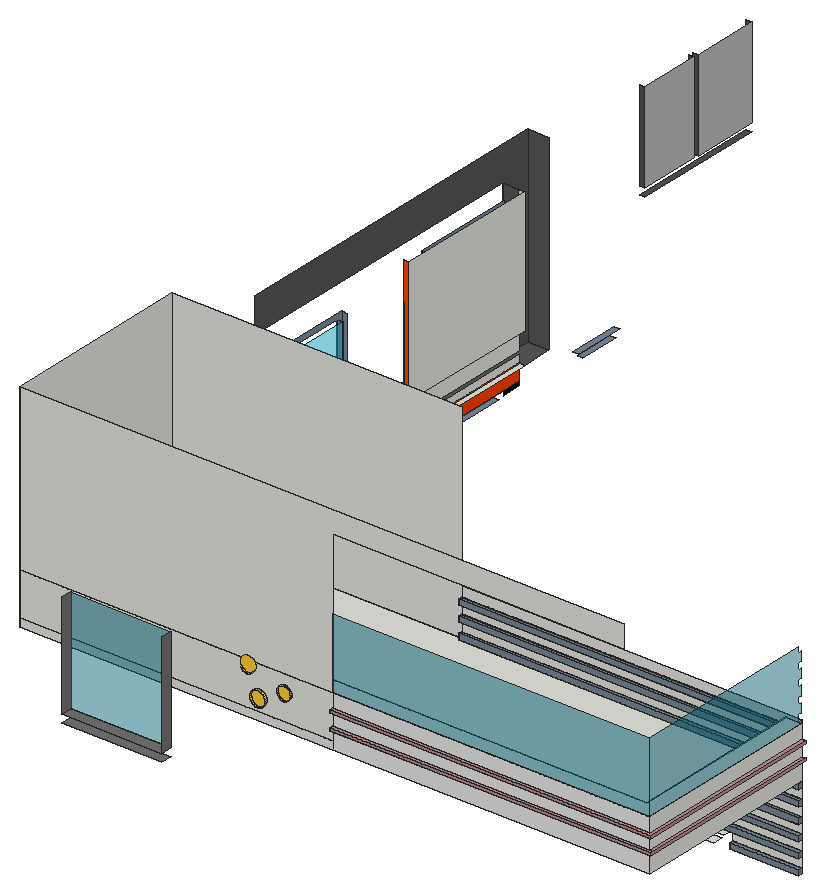
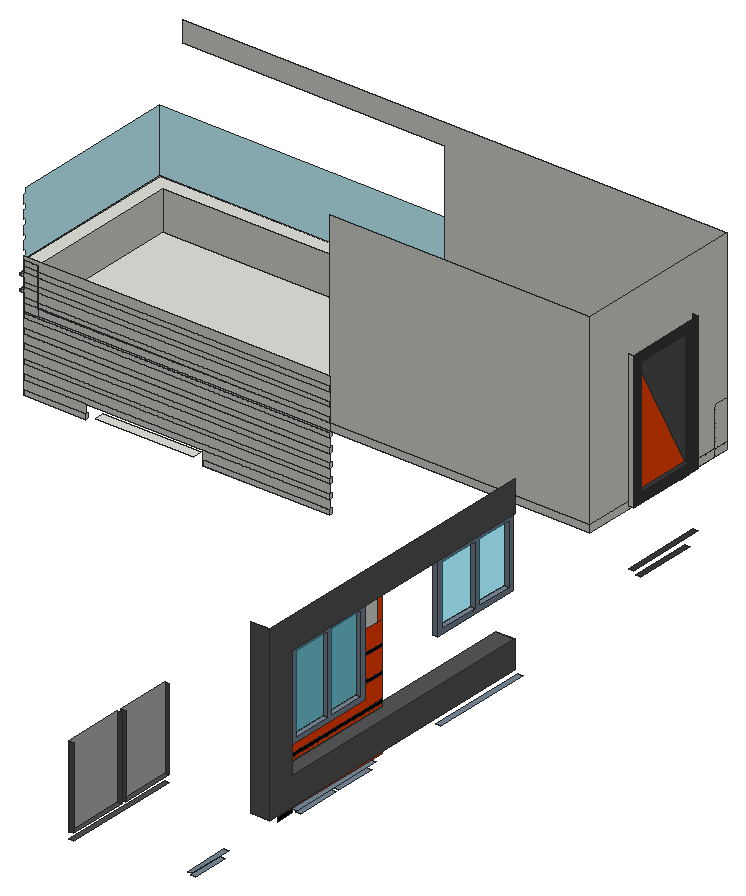
# SketchUp Ruby script. Lengths in inches.
U = 1.inch
M = Sketchup.active_model
def pt(a) = Geom::Point3d.new(a.map { |v| v * U })
def face(e, loops, mat)
  f = e.add_face(loops[0].map { |a| pt(a) })
  loops[1..].each { |l| e.add_face(l.map { |a| pt(a) }).erase! }
  f.material = f.back_material = mat if mat
  f
end
# faces: each face lists its corners as indices into pts; further lists are holes
def faces(e, pts, list, mat = nil) = list.each { |f| face(e, (f[0].is_a?(Array) ? f : [f]).map { |l| l.map { |i| pts[i] } }, mat) }
# xy, xz, yz: faces in a plane at the given z, y or x. An outline is a flat list of corners, or four numbers for a rectangle; further outlines are holes
def ring(l) = l.size == 4 ? [[l[0], l[1]], [l[2], l[1]], [l[2], l[3]], [l[0], l[3]]] : l.each_slice(2).to_a
def flat(e, list, mat, &to3) = list.each { |f| face(e, (f[0].is_a?(Array) ? f : [f]).map { |l| ring(l).map { |u, v| to3.(u, v) } }, mat) }
def xy(e, z, list, mat = nil) = flat(e, list, mat) { |x, y| [x, y, z] }
def xz(e, y, list, mat = nil) = flat(e, list, mat) { |x, z| [x, y, z] }
def yz(e, x, list, mat = nil) = flat(e, list, mat) { |y, z| [x, y, z] }
def lines(e, pts, list) = list.each { |a, b| e.add_line(pt(pts[a]), pt(pts[b])) }
# prism: a flat outline (further loops are holes) pulled along v
def prism(e, loops, v, mat = nil)
  f = face(e, loops, mat); d = Geom::Vector3d.new(v.map { |x| x * U })
  f.pushpull(f.normal.samedirection?(d) ? d.length : -d.length)
end
def box(e, o, s, mat = nil) = prism(e, [[o, [o[0] + s[0], o[1], o[2]], [o[0] + s[0], o[1] + s[1], o[2]], [o[0], o[1] + s[1], o[2]]]], [0, 0, s[2]], mat)
def at(x, y, z, deg = 0) = Geom::Transformation.translation(pt([x, y, z])) * Geom::Transformation.rotation(ORIGIN, Z_AXIS, deg.degrees)
def axes(o, x, y, z) = Geom::Transformation.new([*x, 0, *y, 0, *z, 0, *pt(o).to_a, 1])
def part(name) = M.definitions.add(name)
# library, detail: a bought-in or finely detailed component or shape, given as its bounding box
def library(name, o, s) = part(name).tap { |d| box(d.entities, o, s) }
def detail(e, o, s) = box(e.add_group.entities, o, s)
def put(e, d, t, mat = nil) = e.add_instance(d, t).tap { |i| i.material = mat if mat }
def group(e, t, mat = nil) = e.add_group.tap { |g| g.transformation = t; g.material = mat if mat }.entities
root = M.entities
M.materials.add("[0024_OrangeRed]").color = [255, 69, 0]
M.materials.add("[0110_LightSlateGray]").color = [119, 136, 153]
M.materials.add("[0119_RosyBrown]").color = [188, 143, 143]
M.materials.add("[0135_DarkGray]").color = [81, 81, 81]
M.materials.add("[Color B05]").color = [255, 63, 0]
M.materials.add("[Color D04]").color = [255, 204, 50]
M.materials.add("[Color M05]").color = [114, 114, 114]
M.materials.add("[Color M06]").color = [86, 86, 86]
M.materials.add("[Color M07]").color = [58, 58, 58]
M.materials.add("[Color M09]").color = [0, 0, 0]
M.materials.add("[Mirror 01]").color = [185, 185, 185]
M.materials.add("[Polished Concrete Old]").color = [229, 229, 229]
M.materials.add("[Translucent Glass Tinted]").color = [4, 119, 142]
M.materials["[Translucent Glass Tinted]"].alpha = 0.48
M.materials.add("[Translucent Glass Tinted]1").color = [8, 201, 241]
M.materials["[Translucent Glass Tinted]1"].alpha = 0.48
xy(root,73.4,[[188.34,123.9375,266.69,125.9375],[339.4,123.9375,363.6875,125.9375],[363.6875,123.9375,378,125.9375]],"[0110_LightSlateGray]")
xy(root,74.11,[[15,423.33,18,445.89]],"[0110_LightSlateGray]")
xy(root,74.62,[[15,192.9,18,256.21]],"[0110_LightSlateGray]")
xy(root,75.97,[[272.69,119.9375,333.4,125.9375]])
xy(root,76.125,[[12,313.47,15,338.88],[12,341.11,15,368.75]],"[0110_LightSlateGray]")
xy(root,76.47,[[188.34,123.9375,266.69,125.9375]])
xy(root,76.47,[[339.4,123.9375,378,125.9375]],"[0110_LightSlateGray]")
xy(root,77.11,[[15,420.33,18,448.89]],"[0110_LightSlateGray]")
xy(root,79.125,[[12,310.47,15,371.75]],"[0110_LightSlateGray]")
xy(root,81.97,[[266.69,119.9375,339.4,123.9375],[266.69,123.9375,339.4,125.9375]])
xy(root,81.97,[[188.34,123.9375,266.69,125.9375],[339.4,123.9375,363.6875,125.9375],[363.6875,123.9375,378,125.9375]],"[0110_LightSlateGray]")
xy(root,85.03,[[188.34,123.9375,378,125.9375]],"[0110_LightSlateGray]")
xy(root,88.11,[[15,302.14,18,382.63]])
xy(root,88.11,[[6,209.95,6,399.82,18,399.82,18,382.63,15,382.63,15,302.14,18,302.14,18,209.95]],"[Color M06]")
xy(root,89.01,[[59.9,8,115.9,14]],"[Color M05]")
xy(root,90.53,[[188.34,123.9375,363.6875,125.9375],[363.6875,123.9375,378,125.9375]],"[0110_LightSlateGray]")
xy(root,91.99,[[12,66.99,15,104.86]],"[Color M07]")
xy(root,93.35,[[59.9,8,115.9,14]],"[Color M05]")
xy(root,93.59,[[188.34,123.9375,378,125.9375]],"[0110_LightSlateGray]")
xy(root,97.99,[[12,60.99,15,110.86]],"[Color M07]")
xy(root,99.09,[[188.34,123.9375,363.6875,125.9375],[363.6875,123.9375,378,125.9375]],"[0110_LightSlateGray]")
xy(root,102.16,[[188.34,123.9375,378,125.9375]],"[0110_LightSlateGray]")
xy(root,105.46,[[15,302.36,18,382.63]])
xy(root,105.46,[[6,209.95,18,209.95,18,302.36,15,302.36,15,382.63,6,382.63]],"[Color M06]")
xy(root,107.65,[[188.34,123.9375,363.6875,125.9375],[363.6875,123.9375,378,125.9375]],"[0110_LightSlateGray]")
xy(root,110.72,[[188.34,123.9375,378,125.9375]],"[0110_LightSlateGray]")
xy(root,116.22,[[188.34,123.9375,363.6875,125.9375],[363.6875,123.9375,378,125.9375]],"[0110_LightSlateGray]")
xy(root,117.125,[[12,318.75,15,375.75]],"[0110_LightSlateGray]")
xy(root,119.28,[[188.34,123.9375,378,125.9375]],"[0110_LightSlateGray]")
xy(root,120,[[27,20,378,125.9375]],"[Polished Concrete Old]")
xy(root,120.125,[[12,321.75,15,345.13],[12,347.25,15,372.75]],"[0110_LightSlateGray]")
xy(root,124.4375,[[27,20,201.375,20,188.34,125.9375,27,125.9375]])
xy(root,124.54,[[27,29,369,125.9375]])
xy(root,124.78,[[188.34,123.9375,363.6875,125.9375],[363.6875,123.9375,369,125.9375]])
xy(root,124.92,[[15,200.12,18,258.87]],"[0110_LightSlateGray]")
xy(root,127.84,[[188.34,123.9375,369,125.9375]],"[0110_LightSlateGray]")
xy(root,127.92,[[15,203.12,18,226.79],[15,229.5,18,255.87]],"[0110_LightSlateGray]")
xy(root,130.4,[[201.375,18,201.375,20,378,20,378,125.9375,380,125.9375,380,18]],"[0119_RosyBrown]")
xy(root,131.88,[[201.375,18,380,20],[378,20,380,125.9375]],"[0119_RosyBrown]")
xy(root,132.49,[[12,60.99,15,110.86]])
xy(root,133.34,[[363.6875,123.9375,369,125.9375]])
xy(root,133.34,[[188.34,123.9375,363.6875,125.9375]],"[0110_LightSlateGray]")
xy(root,135.41,[[15,466.73,18,540.73]],"[0135_DarkGray]")
xy(root,136.41,[[188.34,123.9375,369,125.9375]],"[0110_LightSlateGray]")
xy(root,138.49,[[12,66.99,15,104.86]],"[Color M07]")
xy(root,139.21,[[201.375,18,201.375,20,378,20,378,125.9375,380,125.9375,380,18]],"[0119_RosyBrown]")
xy(root,139.68,[[15,466.73,18,500.63],[15,503.73,18,540.73]],"[0135_DarkGray]")
xy(root,140.7,[[201.375,18,380,18,380,125.9375,378,125.9375,378,20,201.375,20]],"[0119_RosyBrown]")
xy(root,141.9,[[363.6875,123.9375,369,125.9375]])
xy(root,141.9,[[188.34,123.9375,363.6875,125.9375]],"[0110_LightSlateGray]")
xy(root,144.97,[[188.34,123.9375,369,125.9375]],"[0110_LightSlateGray]")
xy(root,148.54,[[27,20,378,20,378,125.9375,369,125.9375,369,29,27,29]])
xz(root,11.875,[[181.03,140.83,182.03,140.97,182.97,141.35,183.77,141.97,184.39,142.77,184.77,143.71,184.9,144.71,184.77,145.71,184.39,146.65,183.77,147.45,182.97,148.0625,182.03,148.45,181.03,148.58,180.03,148.45,179.09,148.0625,178.29,147.45,177.67,146.65,177.29,145.71,177.15,144.71,177.29,143.71,177.67,142.77,178.29,141.97,179.09,141.35,180.03,140.97]],"[Color D04]")
xz(root,12.0625,[[160.62,147.68,161.7,147.83,162.71,148.24,163.58,148.91,164.25,149.78,164.67,150.79,164.81,151.87,164.67,152.95,164.25,153.96,163.58,154.83,162.71,155.5,161.7,155.92,160.62,156.06,159.54,155.92,158.53,155.5,157.66,154.83,156.99,153.96,156.58,152.95,156.43,151.87,156.58,150.79,156.99,149.78,157.66,148.91,158.53,148.24,159.54,147.83]],"[Color D04]")
xz(root,12.25,[[166.47,132.54,167.6,132.69,168.65,133.13,169.5625,133.83,170.26,134.73,170.69,135.79,170.84,136.92,170.69,138.05,170.26,139.11,169.5625,140.01,168.65,140.71,167.6,141.14,166.47,141.29,165.33,141.14,164.28,140.71,163.375,140.01,162.68,139.11,162.24,138.05,162.09,136.92,162.24,135.79,162.68,134.73,163.375,133.83,164.28,133.13,165.33,132.69]],"[Color D04]")
xz(root,14,[[59.9,93.35,115.9,151.59]],"[Translucent Glass Tinted]")
xz(root,18,[[201.375,130.4,380,131.88],[201.375,139.21,380,140.7]],"[0119_RosyBrown]")
xz(root,20,[[27,120,201.375,124.4375],[27,124.4375,201.375,148.54],[27,148.54,27,240,363.6875,240,363.6875,227.53,201.375,227.53,201.375,148.54]])
xz(root,20,[[201.375,120,378,130.4],[201.375,131.88,378,139.21],[201.375,140.7,378,148.54]],"[Polished Concrete Old]")
xz(root,20,[[201.375,148.54,378,187.78]],"[Translucent Glass Tinted]")
xz(root,29,[[27,124.54,201.375,148.54],[201.375,124.54,369,148.54]])
xz(root,60.99,[[12,132.49,15,217.37]],"[Color M07]")
xz(root,66.99,[[12,138.49,15,211.37]],"[Color M07]")
xz(root,104.86,[[12,138.49,15,211.37]],"[Color M07]")
xz(root,110.86,[[12,132.49,15,217.37]])
xz(root,123.9375,[[188.34,73.4,266.69,76.47],[339.4,73.4,378,76.47],[188.34,81.97,378,85.03],[188.34,90.53,378,93.59],[188.34,99.09,378,102.16],
  [188.34,107.65,378,110.72],[188.34,116.22,378,119.28],[188.34,124.78,369,127.84],[188.34,133.34,369,136.41],[188.34,141.9,369,144.97]],"[0110_LightSlateGray]")
xz(root,125.9375,[[188.34,73.4,266.69,76.47],[339.4,73.4,378,76.47],[188.34,76.47,266.69,81.97],[339.4,76.47,378,81.97],[188.34,81.97,378,85.03],
  [188.34,85.03,378,90.53],[188.34,90.53,378,93.59],[188.34,93.59,378,99.09],[188.34,99.09,378,102.16],[188.34,102.16,378,107.65],
  [188.34,107.65,378,110.72],[188.34,110.72,378,116.22],[188.34,116.22,378,119.28],[188.34,119.28,378,120],[27,120,188.34,124.4375],
  [188.34,120,369,124.54],[369,120,378,124.78],[27,124.54,188.34,240],[188.34,124.54,369,124.78],[188.34,124.78,369,127.84],
  [369,124.78,378,127.84],[188.34,127.84,369,133.34],[369,127.84,378,133.34],[378,130.4,380,131.88],[188.34,133.34,369,136.41],
  [369,133.34,378,136.41],[188.34,136.41,369,141.9],[369,136.41,378,141.9],[378,139.21,380,140.7],[188.34,141.9,369,144.97],
  [369,141.9,378,144.97],[188.34,144.97,369,144.97,369,148.54,378,148.54,378,150.47,188.34,150.47],[369,144.97,378,148.54]])
xz(root,200.12,[[15,124.92,18,168.42]],"[0110_LightSlateGray]")
xz(root,203.12,[[15,127.92,18,165.42]],"[0110_LightSlateGray]")
xz(root,209.95,[[6,88.11,18,105.46]],"[Color M06]")
xz(root,226.79,[[15,127.92,18,165.42]],"[0110_LightSlateGray]")
xz(root,229.5,[[15,127.92,18,165.42]],"[0110_LightSlateGray]")
xz(root,255.87,[[15,127.92,18,165.42]],"[0110_LightSlateGray]")
xz(root,258.87,[[15,124.92,18,168.42]],"[0110_LightSlateGray]")
xz(root,302.36,[[15,105.46,18,174.92]],"[0024_OrangeRed]")
xz(root,318.75,[[12,117.125,15,171.375]],"[0110_LightSlateGray]")
xz(root,321.75,[[12,120.125,15,168.375]],"[0110_LightSlateGray]")
xz(root,345.13,[[12,120.125,15,168.375]],"[0110_LightSlateGray]")
xz(root,347.25,[[12,120.125,15,168.375]],"[0110_LightSlateGray]")
xz(root,372.75,[[12,120.125,15,168.375]],"[0110_LightSlateGray]")
xz(root,375.75,[[12,117.125,15,171.375]],"[0110_LightSlateGray]")
xz(root,382.63,[[15,105.46,18,174.92]])
xz(root,382.63,[[6,105.46,15,174.92]],"[Color M06]")
xz(root,399.82,[[6,88.11,18,194.23]],"[Color M06]")
xz(root,466.73,[[15,139.68,18,190.1]],"[0135_DarkGray]")
xz(root,500.63,[[15,139.68,18,190.1]],"[0135_DarkGray]")
xz(root,503.73,[[15,139.68,18,190.1]],"[0135_DarkGray]")
xz(root,540.73,[[15,139.68,18,190.1]],"[0135_DarkGray]")
yz(root,6,[[209.95,88.11,209.95,105.46,382.63,105.46,382.63,174.92,209.95,174.92,209.95,194.23,399.82,194.23,399.82,88.11]],"[Color M06]")
yz(root,12,[[[318.75,117.125,375.75,171.375],[347.25,120.125,372.75,168.375],[321.75,120.125,345.13,168.375]]],"[0110_LightSlateGray]")
yz(root,12,[[[60.99,132.49,110.86,217.37],[66.99,138.49,104.86,211.37]]],"[Color M07]")
yz(root,15,[[302.36,88.11,382.63,92.25],[302.36,94.5,382.63,105.46]])
yz(root,15,[[375.75,125.25,382.63,138.375],[66.99,138.49,104.86,211.37,104.86,138.49],[375.75,140.625,382.63,153.75]],"[0024_OrangeRed]")
yz(root,15,[[[200.12,124.92,258.87,168.42],[229.5,127.92,255.87,165.42],[203.12,127.92,226.79,165.42]]],"[0110_LightSlateGray]")
yz(root,15,[[66.99,138.49,66.99,211.37,104.86,211.37]],"[0135_DarkGray]")
yz(root,15,[[302.36,79.125,382.63,88.11],[302.36,105.46,382.63,107.625],[302.36,109.875,302.36,123,318.75,123,318.75,117.125,375.75,117.125,375.75,123,382.63,123,382.63,109.875],[302.36,125.25,318.75,138.375],[302.36,140.625,318.75,153.75]],"[Color B05]")
yz(root,15,[[371.75,76.875,382.63,79.125],[302.36,107.625,382.63,109.875],[302.36,123,318.75,125.25],[375.75,123,382.63,125.25],[302.36,138.375,318.75,140.625],
  [375.75,138.375,382.63,140.625]],"[Color M09]")
yz(root,15,[[321.75,120.125,345.13,168.375],[347.25,120.125,372.75,168.375]],"[Translucent Glass Tinted]1")
yz(root,18,[[302.36,105.46,382.63,174.92]])
yz(root,18,[[466.73,139.68,500.63,190.1],[503.73,139.68,540.73,190.1]],"[Mirror 01]")
yz(root,18,[[203.12,127.92,226.79,165.42],[229.5,127.92,255.87,165.42]],"[Translucent Glass Tinted]1")
yz(root,27,[[20,120,29,124.4375],[29,120,125.9375,124.4375],[20,124.4375,29,148.54],[29,124.54,125.9375,124.54,125.9375,240,20,240,20,148.54,29,148.54]])
yz(root,59.9,[[8,93.35,14,151.59]],"[Color M05]")
yz(root,115.9,[[8,93.35,14,151.59]],"[Color M05]")
yz(root,188.34,[[123.9375,73.4,125.9375,76.47],[123.9375,81.97,125.9375,85.03],[123.9375,90.53,125.9375,93.59],[123.9375,99.09,125.9375,102.16],[123.9375,107.65,125.9375,110.72],
  [123.9375,116.22,125.9375,119.28]])
yz(root,188.34,[[123.9375,124.78,125.9375,127.84],[123.9375,133.34,125.9375,136.41],[123.9375,141.9,125.9375,144.97]],"[0110_LightSlateGray]")
yz(root,201.375,[[18,130.4,20,131.88],[18,139.21,20,140.7]])
yz(root,266.69,[[123.9375,73.4,125.9375,76.47]])
yz(root,339.4,[[123.9375,73.4,125.9375,76.47]])
yz(root,369,[[29,124.54,29,148.54,125.9375,148.54,125.9375,144.97,123.9375,144.97,123.9375,141.9,125.9375,141.9,125.9375,136.41,123.9375,136.41,123.9375,133.34,125.9375,133.34,125.9375,127.84,123.9375,127.84,123.9375,124.78,125.9375,124.78,125.9375,124.54],[123.9375,124.78,125.9375,127.84],[123.9375,133.34,125.9375,136.41],[123.9375,141.9,125.9375,144.97]])
yz(root,378,[[20,120,125.9375,130.4],[20,131.88,125.9375,139.21],[20,140.7,125.9375,148.54]])
yz(root,378,[[123.9375,73.4,125.9375,76.47],[123.9375,81.97,125.9375,85.03],[123.9375,90.53,125.9375,93.59],[123.9375,99.09,125.9375,102.16],[123.9375,107.65,125.9375,110.72],
  [123.9375,116.22,125.9375,119.28]],"[0110_LightSlateGray]")
yz(root,378,[[20,148.54,125.9375,148.54,125.9375,150.47,123.9375,150.47,123.9375,153.53,125.9375,153.53,125.9375,159.03,123.9375,159.03,123.9375,162.09,125.9375,162.09,125.9375,167.59,123.9375,167.59,123.9375,170.66,125.9375,170.66,125.9375,176.15,123.9375,176.15,123.9375,179.22,125.9375,179.22,125.9375,184.72,123.9375,184.72,123.9375,187.78,20,187.78]],"[Translucent Glass Tinted]")
yz(root,380,[[18,130.4,125.9375,131.88],[18,139.21,125.9375,140.7]],"[0119_RosyBrown]")
p = [[165.33,11,132.69],[166.47,11,132.54],[166.47,12.25,132.54],[165.33,12.25,132.69],[167.6,11,132.69],[167.6,12.25,132.69],
  [164.28,11,133.13],[164.28,12.25,133.13],[168.65,11,133.13],[168.65,12.25,133.13],[163.375,11,133.83],[163.375,12.25,133.83],
  [169.5625,11,133.83],[169.5625,12.25,133.83],[162.68,11,134.73],[162.68,12.25,134.73],[170.26,11,134.73],[170.26,12.25,134.73],
  [162.24,11,135.79],[162.24,12.25,135.79],[170.69,11,135.79],[170.69,12.25,135.79],[162.09,11,136.92],[162.09,12.25,136.92],
  [170.84,11,136.92],[170.84,12.25,136.92],[162.24,11,138.05],[162.24,12.25,138.05],[170.69,11,138.05],[170.69,12.25,138.05],
  [162.68,11,139.11],[162.68,12.25,139.11],[170.26,11,139.11],[170.26,12.25,139.11],[163.375,11,140.01],[163.375,12.25,140.01],
  [169.5625,11,140.01],[169.5625,12.25,140.01],[164.28,11,140.71],[164.28,12.25,140.71],[168.65,11,140.71],[168.65,12.25,140.71],
  [165.33,11,141.14],[165.33,12.25,141.14],[167.6,11,141.14],[167.6,12.25,141.14],[180.03,11,140.97],[181.03,11,140.83],
  [181.03,11.875,140.83],[180.03,11.875,140.97],[182.03,11,140.97],[182.03,11.875,140.97],[179.09,11,141.35],[179.09,11.875,141.35],
  [182.97,11,141.35],[182.97,11.875,141.35],[166.47,11,141.29],[166.47,12.25,141.29],[178.29,11,141.97],[178.29,11.875,141.97],
  [183.77,11,141.97],[183.77,11.875,141.97],[177.67,11,142.77],[177.67,11.875,142.77],[184.39,11,142.77],[184.39,11.875,142.77],
  [177.29,11,143.71],[177.29,11.875,143.71],[184.77,11,143.71],[184.77,11.875,143.71],[177.15,11,144.71],[177.15,11.875,144.71],
  [184.9,11,144.71],[184.9,11.875,144.71],[177.29,11,145.71],[177.29,11.875,145.71],[184.77,11,145.71],[184.77,11.875,145.71],
  [177.67,11,146.65],[177.67,11.875,146.65],[184.39,11,146.65],[184.39,11.875,146.65],[178.29,11,147.45],[178.29,11.875,147.45],
  [183.77,11,147.45],[183.77,11.875,147.45],[179.09,11,148.0625],[179.09,11.875,148.0625],[182.97,11,148.0625],[182.97,11.875,148.0625],
  [159.54,11,147.83],[160.62,11,147.68],[160.62,12.0625,147.68],[159.54,12.0625,147.83],[161.7,11,147.83],[161.7,12.0625,147.83],
  [158.53,11,148.24],[158.53,12.0625,148.24],[162.71,11,148.24],[162.71,12.0625,148.24],[180.03,11,148.45],[180.03,11.875,148.45],
  [182.03,11,148.45],[182.03,11.875,148.45],[157.66,11,148.91],[157.66,12.0625,148.91],[163.58,11,148.91],[163.58,12.0625,148.91],
  [181.03,11,148.58],[181.03,11.875,148.58],[156.99,11,149.78],[156.99,12.0625,149.78],[164.25,11,149.78],[164.25,12.0625,149.78]]
faces(root,p,[[0,1,2,3],[1,4,5,2],[6,0,3,7],[4,8,9,5],[10,6,7,11],[8,12,13,9],[14,10,11,15],[12,16,17,13],
  [18,14,15,19],[16,20,21,17],[22,18,19,23],[20,24,25,21],[26,22,23,27],[24,28,29,25],[30,26,27,31],[28,32,33,29],
  [34,30,31,35],[32,36,37,33],[38,34,35,39],[36,40,41,37],[42,38,39,43],[40,44,45,41],[46,47,48,49],[47,50,51,48],
  [52,46,49,53],[50,54,55,51],[56,42,43,57],[44,56,57,45],[58,52,53,59],[54,60,61,55],[62,58,59,63],[60,64,65,61],
  [66,62,63,67],[64,68,69,65],[70,66,67,71],[68,72,73,69],[74,70,71,75],[72,76,77,73],[78,74,75,79],[76,80,81,77],
  [82,78,79,83],[80,84,85,81],[86,82,83,87],[84,88,89,85],[90,91,92,93],[91,94,95,92],[96,90,93,97],[94,98,99,95],
  [100,86,87,101],[88,102,103,89],[104,96,97,105],[98,106,107,99],[108,100,101,109],[102,108,109,103],[110,104,105,111],[106,112,113,107]],"[Color D04]")
